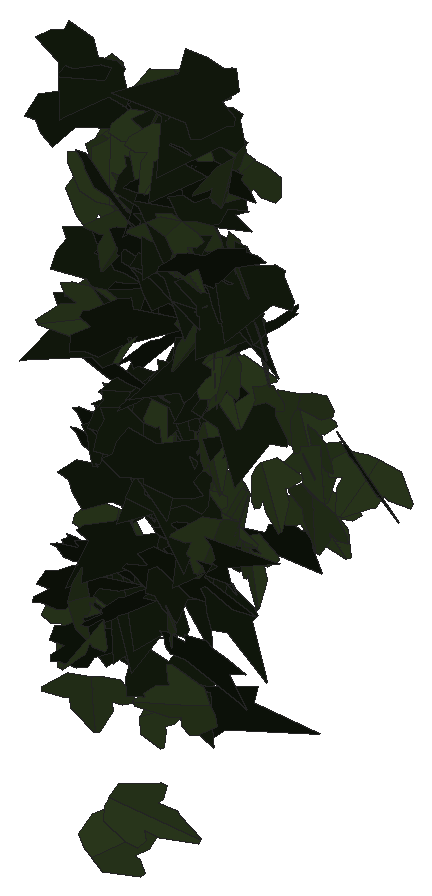
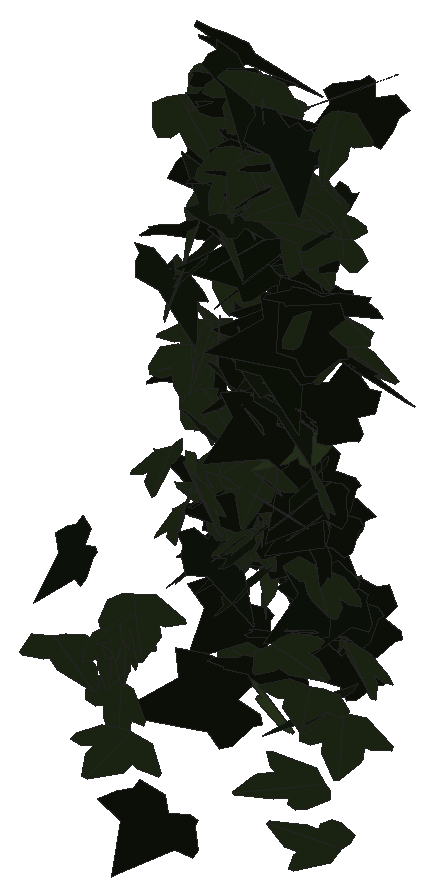
# SketchUp Ruby script. Lengths in inches.
U = 1.inch
M = Sketchup.active_model
def pt(a) = Geom::Point3d.new(a.map { |v| v * U })
def face(e, loops, mat)
  f = e.add_face(loops[0].map { |a| pt(a) })
  loops[1..].each { |l| e.add_face(l.map { |a| pt(a) }).erase! }
  f.material = f.back_material = mat if mat
  f
end
# faces: each face lists its corners as indices into pts; further lists are holes
def faces(e, pts, list, mat = nil) = list.each { |f| face(e, (f[0].is_a?(Array) ? f : [f]).map { |l| l.map { |i| pts[i] } }, mat) }
# xy, xz, yz: faces in a plane at the given z, y or x. An outline is a flat list of corners, or four numbers for a rectangle; further outlines are holes
def ring(l) = l.size == 4 ? [[l[0], l[1]], [l[2], l[1]], [l[2], l[3]], [l[0], l[3]]] : l.each_slice(2).to_a
def flat(e, list, mat, &to3) = list.each { |f| face(e, (f[0].is_a?(Array) ? f : [f]).map { |l| ring(l).map { |u, v| to3.(u, v) } }, mat) }
def xy(e, z, list, mat = nil) = flat(e, list, mat) { |x, y| [x, y, z] }
def xz(e, y, list, mat = nil) = flat(e, list, mat) { |x, z| [x, y, z] }
def yz(e, x, list, mat = nil) = flat(e, list, mat) { |y, z| [x, y, z] }
def lines(e, pts, list) = list.each { |a, b| e.add_line(pt(pts[a]), pt(pts[b])) }
# prism: a flat outline (further loops are holes) pulled along v
def prism(e, loops, v, mat = nil)
  f = face(e, loops, mat); d = Geom::Vector3d.new(v.map { |x| x * U })
  f.pushpull(f.normal.samedirection?(d) ? d.length : -d.length)
end
def box(e, o, s, mat = nil) = prism(e, [[o, [o[0] + s[0], o[1], o[2]], [o[0] + s[0], o[1] + s[1], o[2]], [o[0], o[1] + s[1], o[2]]]], [0, 0, s[2]], mat)
def at(x, y, z, deg = 0) = Geom::Transformation.translation(pt([x, y, z])) * Geom::Transformation.rotation(ORIGIN, Z_AXIS, deg.degrees)
def axes(o, x, y, z) = Geom::Transformation.new([*x, 0, *y, 0, *z, 0, *pt(o).to_a, 1])
def part(name) = M.definitions.add(name)
# library, detail: a bought-in or finely detailed component or shape, given as its bounding box
def library(name, o, s) = part(name).tap { |d| box(d.entities, o, s) }
def detail(e, o, s) = box(e.add_group.entities, o, s)
def put(e, d, t, mat = nil) = e.add_instance(d, t).tap { |i| i.material = mat if mat }
def group(e, t, mat = nil) = e.add_group.tap { |g| g.transformation = t; g.material = mat if mat }.entities
root = M.entities
M.materials.add("1026 AP 7946 SUNNY SIDE UP").color = [254, 231, 186]
M.materials.add("efeu1").color = [18, 25, 13]
M.materials.add("efeu2").color = [43, 57, 29]
c1 = part("ivyleaf_9")
p = [[1.54,2.16,1.25],[1.36,2.04,1.19],[-0.21,0.99,0.68],[-0.71,1.11,0.82],[-0.85,0.86,0.67],[-0.8,0.17,0.21],
  [-0.9,-0.01,0.1],[-0.67,-0.16,-0.02],[-0.08,-0.08,-0.05],[-0.03,-0.6,-0.4],[0.65,-0.88,-0.66],[0.83,-0.6,-0.49],
  [1.29,-0.42,-0.43],[1.8125,-0.07,-0.26],[1.21,0.44,0.15]]
faces(c1.entities,p,[[0,1,2,3,4,5,6,7,8,9,10,11,12,13,14]],"efeu1")
c2 = part("ivyleaf_10")
p = [[0,0.5,-0.03],[-0.0625,2.02,-0.43],[-0.19,2.01,-0.46],[-0.54,1.05,-0.29],[-0.52,0.625,-0.18],[-0.83,0.76,-0.28],
  [-1.16,0.64,-0.33],[-1.15,0.33,-0.24],[-0.77,-0.39,0.02],[-0.3,-0.51,0.16],[0.04,-0.48,0.23],[-0.02,2.01,-0.4375],
  [-0.06,2.01,-0.43],[0.04,-0.49,0.23],[0.67,-0.49,0.14],[1.38,0.36,-0.2],[1.375,0.51,-0.24],[0.81,0.65,-0.19],
  [0.62,0.59,-0.15],[0.6,1.09,-0.28],[0.5,1.23,-0.31]]
faces(c2.entities,p,[[0,1,2,3,4,5,6,7,8,9,10],[11,12,0,13,14,15,16,17,18,19,20]],"efeu2")
put(root,c1,axes([137.95,216.12,282.3],[0.42872,0.18972,0.0152],[0.02688,-0.00063,-0.34203],[-0.29788,0.27299,-0.00899]),"1026 AP 7946 SUNNY SIDE UP")
put(root,c1,axes([138.37,212.3,287.125],[-0.53188,0.04679,0.02114],[-0.04146,-0.04424,-0.34865],[-0.06861,-0.33596,0.04682]),"1026 AP 7946 SUNNY SIDE UP")
put(root,c2,axes([138.14,212.36,281.83],[-0.43427,-0.18901,-0.01024],[0.03781,-0.0195,-0.34353],[0.29512,-0.27563,0.02895]),"1026 AP 7946 SUNNY SIDE UP")
put(root,c2,axes([138.07,212.53,290.51],[-0.12663,-0.33819,-0.11167],[0.13132,0.08802,-0.35258],[0.54182,-0.10037,0.05935]),"1026 AP 7946 SUNNY SIDE UP")
put(root,c2,axes([138.08,212.2,282.89],[0.50514,-0.1536,0.01031],[-0.0055,-0.03245,-0.36566],[0.24207,0.3198,-0.02983]),"1026 AP 7946 SUNNY SIDE UP")
put(root,c1,axes([137.84,211.95,283.31],[0.26338,0.12076,0.27193],[0.34927,0.14163,-0.21168],[-0.29229,0.27805,-0.00792]),"1026 AP 7946 SUNNY SIDE UP")
put(root,c2,axes([137.98,213.19,282.72],[0.45525,0.13542,0.05238],[0.07469,0.01662,-0.32914],[-0.21439,0.29335,-0.00345]),"1026 AP 7946 SUNNY SIDE UP")
put(root,c2,axes([138.48,212.25,287.32],[0.34135,-0.05933,-0.31556],[-0.48308,0.02202,-0.22883],[0.08247,0.37451,-0.03428]),"1026 AP 7946 SUNNY SIDE UP")
put(root,c2,axes([138.14,212.86,285.62],[0.31499,-0.27005,0.01951],[0.03733,-0.00785,-0.34612],[0.42421,0.20121,0.01597]),"1026 AP 7946 SUNNY SIDE UP")
put(root,c1,axes([137.91,212.79,282.46],[0.31932,-0.22127,-0.13605],[-0.01575,0.15977,-0.2935],[0.40387,0.18118,0.09612]),"1026 AP 7946 SUNNY SIDE UP")
put(root,c1,axes([137.92,212.73,285.13],[0.52286,-0.01739,0.00805],[0.01101,-0.01733,-0.34269],[0.02794,0.33217,-0.01551]),"1026 AP 7946 SUNNY SIDE UP")
put(root,c2,axes([138.32,211.83,283.34],[-0.07815,0.13055,0.37213],[-0.2649,0.31909,-0.14111],[-0.54154,-0.17493,0.01532]),"1026 AP 7946 SUNNY SIDE UP")
put(root,c1,axes([138.15,212.42,283.77],[0.46242,0.10446,-0.11005],[-0.18167,0.00744,-0.31837],[-0.15001,0.313,0.04633]),"1026 AP 7946 SUNNY SIDE UP")
put(root,c1,axes([137.93,212.95,284.77],[0.03313,-0.03198,-0.33744],[0.4924,-0.09841,0.03009],[-0.15823,-0.31293,0.02299]),"1026 AP 7946 SUNNY SIDE UP")
put(root,c1,axes([138.18,212.37,290.85],[-0.24947,-0.28167,0.17286],[-0.01574,-0.18386,-0.32571],[0.51658,-0.14163,0.07356]),"1026 AP 7946 SUNNY SIDE UP")
put(root,c1,axes([137.97,212.4,283.72],[0.53065,0.096,0.08069],[0.10353,0.05169,-0.35975],[-0.1644,0.34245,0.03389]),"1026 AP 7946 SUNNY SIDE UP")
put(root,c1,axes([138.1,211.8125,290.58],[0.05421,-0.04347,-0.40499],[-0.10373,0.3882,-0.04795],[0.61281,0.06956,0.02771]),"1026 AP 7946 SUNNY SIDE UP")
put(root,c1,axes([137.8125,212.54,286.48],[0.30203,-0.16447,0.24232],[0.32031,-0.12285,-0.25956],[0.31963,0.27852,0.03113]),"1026 AP 7946 SUNNY SIDE UP")
put(root,c1,axes([138.04,212.86,285.14],[0.17389,-0.31256,-0.0502],[-0.00105,0.04951,-0.34088],[0.49698,0.10946,0.01684]),"1026 AP 7946 SUNNY SIDE UP")
put(root,c2,axes([138.22,212.67,284.09],[0.50889,-0.04895,-0.00527],[-0.00167,0.02524,-0.33609],[0.07733,0.32269,0.02743]),"1026 AP 7946 SUNNY SIDE UP")
put(root,c2,axes([138.32,212.57,287.58],[-0.33299,-0.27512,-0.01974],[0.04867,-0.00168,-0.35671],[0.43074,-0.2125,0.02505]),"1026 AP 7946 SUNNY SIDE UP")
put(root,c2,axes([138.45,213.16,283.18],[0.28779,0.15624,-0.22384],[-0.2585,-0.14343,-0.24874],[-0.33349,0.24601,-0.00036]),"1026 AP 7946 SUNNY SIDE UP")
put(root,c1,axes([138.09,211.94,282.59],[0.21475,0.11579,0.29698],[0.39679,0.1411,-0.18114],[-0.28327,0.28543,-0.02858]),"1026 AP 7946 SUNNY SIDE UP")
put(root,c1,axes([138.12,212.58,285.59],[0.52452,0.03111,0.03478],[0.05797,-0.03616,-0.34298],[-0.04267,0.33331,-0.03846]),"1026 AP 7946 SUNNY SIDE UP")
put(root,c1,axes([138.22,212.71,285.45],[0.52771,0.03995,-0.05944],[-0.0825,-0.046,-0.34613],[-0.07372,0.33745,-0.03811]),"1026 AP 7946 SUNNY SIDE UP")
put(root,c2,axes([138.39,212.41,289.0625],[0.61396,0.03855,0.04165],[-0.0709,0.05154,0.40045],[0.05144,-0.38912,0.05483]),"1026 AP 7946 SUNNY SIDE UP")
put(root,c1,axes([138.25,212.61,288.05],[-0.25066,-0.28804,-0.17007],[0.19697,0.11548,-0.33484],[0.48207,-0.19696,0.04838]),"1026 AP 7946 SUNNY SIDE UP")
put(root,c2,axes([138.03,212.48,288.91],[0.29702,-0.00979,0.32478],[0.49582,-0.00506,-0.1948],[0.01473,0.36753,0.00812]),"1026 AP 7946 SUNNY SIDE UP")
put(root,c1,axes([138.16,212.51,289.15],[0.26268,-0.29587,0.08312],[0.07745,-0.06673,-0.35028],[0.47667,0.17389,0.01111]),"1026 AP 7946 SUNNY SIDE UP")
put(root,c1,axes([138.31,212.92,285.22],[0.07404,-0.32159,0.06721],[0.00653,-0.06716,-0.33518],[0.51651,0.04695,-0.0054]),"1026 AP 7946 SUNNY SIDE UP")
put(root,c1,axes([138.68,212.74,290.34],[0.03034,0.35732,0.01618],[0.00274,0.0136,-0.36856],[-0.56225,0.01935,-0.00092]),"1026 AP 7946 SUNNY SIDE UP")
put(root,c2,axes([138.67,212.44,288.64],[-0.15481,-0.30808,0.14282],[-0.02385,-0.14204,-0.33291],[0.53181,-0.09605,0.02665]),"1026 AP 7946 SUNNY SIDE UP")
put(root,c1,axes([138.32,212.36,285.03],[-0.04851,-0.07724,-0.34935],[0.21188,0.31072,-0.08383],[0.50343,-0.13821,0.00162]),"1026 AP 7946 SUNNY SIDE UP")
put(root,c2,axes([138.32,212.69,289.54],[-0.34296,-0.11144,-0.30954],[0.45818,0.08049,-0.24872],[0.2075,-0.36193,0.03757]),"1026 AP 7946 SUNNY SIDE UP")
put(root,c1,axes([138.34,212.69,285.49],[0.35028,-0.24757,0.03355],[0.02972,-0.02869,-0.34323],[0.39181,0.22351,-0.00396]),"1026 AP 7946 SUNNY SIDE UP")
put(root,c1,axes([138.18,212.66,287.61],[0.50767,-0.04597,0.21665],[0.3158,-0.07338,-0.3342],[0.12292,0.3784,-0.03616]),"1026 AP 7946 SUNNY SIDE UP")
put(root,c1,axes([138.86,212.28,284.25],[0.07539,0.13523,-0.32928],[-0.11447,-0.31236,-0.14887],[-0.53472,0.08593,-0.01456]),"1026 AP 7946 SUNNY SIDE UP")
put(root,c2,axes([138.23,212.6875,289.01],[-0.06901,-0.02114,-0.39221],[0.58304,-0.09117,-0.03936],[-0.13894,-0.37211,0.02962]),"1026 AP 7946 SUNNY SIDE UP")
put(root,c1,axes([138.61,212.78,283.04],[-0.12573,-0.30723,0.0906],[-0.00156,-0.09221,-0.32684],[0.50325,-0.07704,0.02162]),"1026 AP 7946 SUNNY SIDE UP")
put(root,c1,axes([138.625,212.01,283.21],[0.23759,0.23325,0.22563],[0.16411,0.19148,-0.28488],[-0.47408,0.18318,0.01446]),"1026 AP 7946 SUNNY SIDE UP")
put(root,c2,axes([138.45,212.61,285.91],[0.37904,-0.2208,-0.07577],[0.31094,0.24967,-0.10484],[0.19178,0.03159,0.31974]),"1026 AP 7946 SUNNY SIDE UP")
put(root,c1,axes([138.75,212.77,283.14],[-0.3728,-0.22969,0.01212],[0.07047,-0.06452,-0.33095],[0.35482,-0.22852,0.07846]),"1026 AP 7946 SUNNY SIDE UP")
put(root,c1,axes([138.99,212.45,286.36],[-0.08541,0.32737,0.07438],[-0.07451,0.06302,-0.33952],[-0.52121,-0.06266,0.03635]),"1026 AP 7946 SUNNY SIDE UP")
put(root,c2,axes([138.83,215.62,284.72],[-0.35815,-0.23538,0.02415],[-0.00161,-0.03342,-0.33683],[0.37215,-0.22667,0.02179]),"1026 AP 7946 SUNNY SIDE UP")
put(root,c1,axes([138.45,212.56,287.36],[0.37956,0.12288,0.2599],[0.37019,0.09073,-0.27782],[-0.2383,0.33665,-0.01762]),"1026 AP 7946 SUNNY SIDE UP")
put(root,c1,axes([138.58,211.875,287.36],[0.1403,0.19253,-0.32],[0.05905,0.31433,0.21292],[0.57306,-0.07952,0.05641]),"1026 AP 7946 SUNNY SIDE UP")
put(root,c2,axes([138.72,216.03,283.02],[-0.41945,-0.14449,-0.14944],[0.26608,-0.02368,-0.29809],[0.17963,-0.30233,0.09259]),"1026 AP 7946 SUNNY SIDE UP")
put(root,c2,axes([138.625,212.01,279.82],[0.2186,0.09048,-0.3152],[0.3582,0.20632,0.17041],[0.35236,-0.26587,0.0223]),"1026 AP 7946 SUNNY SIDE UP")
put(root,c2,axes([138.91,212.98,285.42],[0.13341,0.25701,0.2001],[-0.0959,0.20864,-0.25769],[-0.49598,0.02878,0.10365]),"1026 AP 7946 SUNNY SIDE UP")
put(root,c1,axes([139.08,212.54,287.05],[-0.02278,0.3425,-0.06686],[0.01378,-0.06652,-0.3535],[-0.54854,-0.0159,-0.0061]),"1026 AP 7946 SUNNY SIDE UP")
put(root,c1,axes([138.82,212.51,285.95],[-0.16955,-0.30808,-0.09451],[0.05409,0.08329,-0.33574],[0.50176,-0.11309,0.00426]),"1026 AP 7946 SUNNY SIDE UP")
put(root,c2,axes([139.03,215.64,284.27],[-0.38712,0.21722,0.02043],[-0.09839,-0.04354,-0.3298],[-0.32838,-0.24303,0.07474]),"1026 AP 7946 SUNNY SIDE UP")
put(root,c1,axes([138.85,212.84,286.11],[0.2777,0.20587,0.20723],[0.21585,0.14562,-0.27848],[-0.39633,0.22356,-0.00647]),"1026 AP 7946 SUNNY SIDE UP")
put(root,c1,axes([139.09,212.99,285.125],[-0.47718,-0.06982,-0.11358],[0.19907,-0.09355,-0.29958],[0.04758,-0.30889,0.11434]),"1026 AP 7946 SUNNY SIDE UP")
put(root,c2,axes([139.21,212.78,285.32],[-0.48748,0.01167,0.12091],[-0.18501,-0.05053,-0.31549],[0.01118,-0.3276,0.05101]),"1026 AP 7946 SUNNY SIDE UP")
put(root,c1,axes([139.04,212.625,286.23],[-0.45145,-0.13408,-0.12],[0.19588,0.00382,-0.32292],[0.19797,-0.30953,0.04585]),"1026 AP 7946 SUNNY SIDE UP")
put(root,c2,axes([138.97,215.58,284.48],[0.01954,0.32821,-0.01036],[-0.00123,-0.0119,-0.33843],[-0.51641,0.01245,0.00041]),"1026 AP 7946 SUNNY SIDE UP")
put(root,c2,axes([139.0625,212.67,290.4],[0.14061,-0.3497,-0.01859],[0.06647,0.02724,-0.36843],[0.54641,0.08667,0.0496]),"1026 AP 7946 SUNNY SIDE UP")
put(root,c2,axes([139.17,215.56,283.35],[-0.47317,0.14296,0.05262],[-0.09923,-0.01661,-0.34062],[-0.21663,-0.30464,0.04109]),"1026 AP 7946 SUNNY SIDE UP")
put(root,c2,axes([139.04,212.72,285.86],[0.2255,0.29723,-0.03634],[-0.00697,-0.03887,-0.33996],[-0.47092,0.14291,-0.01237]),"1026 AP 7946 SUNNY SIDE UP")
put(root,c1,axes([138.64,212.36,288.18],[0.24456,-0.05448,0.33598],[0.48034,-0.11514,-0.17041],[0.20022,0.34278,-0.00156]),"1026 AP 7946 SUNNY SIDE UP")
put(root,c1,axes([139.49,212.82,286.11],[-0.10643,-0.13238,-0.31536],[-0.27789,-0.24976,0.15044],[-0.44346,0.18828,-0.01858]),"1026 AP 7946 SUNNY SIDE UP")
put(root,c1,axes([138.98,212.36,285.83],[-0.10527,-0.34112,-0.10654],[0.07399,0.09387,-0.35649],[0.55469,-0.07726,0.02733]),"1026 AP 7946 SUNNY SIDE UP")
put(root,c1,axes([139.42,212.62,286.78],[-0.37173,0.2263,-0.09427],[0.04104,-0.10497,-0.33286],[-0.3824,-0.23126,0.05592]),"1026 AP 7946 SUNNY SIDE UP")
put(root,c2,axes([139.15,212.36,290.16],[0.55968,-0.02919,-0.00552],[-0.01155,-0.02621,-0.36704],[0.04516,0.35501,-0.02545]),"1026 AP 7946 SUNNY SIDE UP")
put(root,c2,axes([139.17,212.71,284.38],[-0.04591,0.28419,-0.1655],[0.0064,-0.16258,-0.29505],[-0.51453,-0.02738,0.0111]),"1026 AP 7946 SUNNY SIDE UP")
put(root,c1,axes([139.08,212.52,289.31],[-0.04327,-0.35443,0.02912],[-0.0005,-0.03035,-0.3664],[0.55933,-0.02744,0.00192]),"1026 AP 7946 SUNNY SIDE UP")
put(root,c2,axes([139.22,215.56,284.12],[-0.23275,-0.29253,-0.01229],[0.11378,-0.02541,-0.32869],[0.44597,-0.14618,0.07744]),"1026 AP 7946 SUNNY SIDE UP")
put(root,c2,axes([139.33,212.66,289.47],[-0.2041,-0.31445,0.09645],[-0.01348,-0.09931,-0.34977],[0.51652,-0.12684,0.02898]),"1026 AP 7946 SUNNY SIDE UP")
put(root,c2,axes([139.19,212.875,284.45],[0.12463,0.31723,-0.0542],[-0.00447,-0.05534,-0.337],[-0.50607,0.07861,-0.01037]),"1026 AP 7946 SUNNY SIDE UP")
put(root,c1,axes([139.48,212.47,285.36],[-0.49738,-0.10483,0.00487],[0.00798,-0.03214,-0.34189],[0.16486,-0.31472,0.03123]),"1026 AP 7946 SUNNY SIDE UP")
put(root,c2,axes([139.14,212.59,286.07],[0.01346,-0.31323,0.15881],[0.29861,-0.12685,-0.27398],[0.46209,0.09109,0.17243]),"1026 AP 7946 SUNNY SIDE UP")
put(root,c1,axes([139.11,212.44,288.21],[0.24839,-0.25169,-0.19586],[-0.08118,0.18754,-0.30113],[0.48791,0.15933,0.04961]),"1026 AP 7946 SUNNY SIDE UP")
put(root,c2,axes([139.04,212.47,281.69],[0.15798,-0.26625,-0.18959],[0.28173,-0.11301,0.27077],[-0.42221,-0.17503,0.10974]),"1026 AP 7946 SUNNY SIDE UP")
put(root,c2,axes([139.27,212.71,290.75],[-0.47222,-0.18249,-0.08389],[0.18001,-0.03877,-0.35011],[0.25674,-0.30846,0.09118]),"1026 AP 7946 SUNNY SIDE UP")
put(root,c1,axes([139.31,212.59,288.93],[-0.23888,-0.29224,0.12369],[-0.03385,-0.12516,-0.33798],[0.49663,-0.1491,0.03645]),"1026 AP 7946 SUNNY SIDE UP")
put(root,c2,axes([139,211.99,280.55],[0.13058,0.10916,0.33207],[0.37123,0.21961,-0.13826],[-0.38412,0.24934,-0.02074]),"1026 AP 7946 SUNNY SIDE UP")
put(root,c1,axes([139.52,212.38,289.59],[0.00696,0.25924,-0.284],[-0.0102,-0.27708,-0.26872],[-0.59663,0.00776,0.00128]),"1026 AP 7946 SUNNY SIDE UP")
put(root,c2,axes([139.61,212.62,284.46],[-0.44664,-0.01544,0.1887],[-0.26993,-0.09869,-0.28326],[0.10373,-0.32331,0.07538]),"1026 AP 7946 SUNNY SIDE UP")
put(root,c1,axes([139.18,212.95,284.48],[0.09888,-0.32337,-0.01361],[-0.0212,0.00896,-0.33912],[0.50835,0.06327,-0.01149]),"1026 AP 7946 SUNNY SIDE UP")
put(root,c1,axes([139.8,212.56,290],[-0.06682,0.05866,0.3661],[-0.5158,0.14066,-0.06357],[-0.23262,-0.32874,0.03579]),"1026 AP 7946 SUNNY SIDE UP")
put(root,c1,axes([139.14,212.88,284.43],[0.27869,-0.28014,-0.00628],[0.02396,0.01496,-0.34074],[0.43989,0.17666,0.02253]),"1026 AP 7946 SUNNY SIDE UP")
put(root,c1,axes([139.01,212.69,284.69],[0.11314,-0.00175,-0.34027],[0.40087,0.2152,0.0573],[0.33018,-0.26068,0.04702]),"1026 AP 7946 SUNNY SIDE UP")
put(root,c1,axes([139.11,212.55,288.09],[-0.02082,-0.31941,0.16766],[0.27102,-0.15013,-0.2868],[0.49572,0.06867,0.16384]),"1026 AP 7946 SUNNY SIDE UP")
put(root,c2,axes([139.2,212.83,285.875],[-0.06909,0.01699,-0.34545],[0.23374,-0.30235,-0.0376],[-0.47354,-0.15172,0.03184]),"1026 AP 7946 SUNNY SIDE UP")
put(root,c1,axes([139.59,212.45,290.67],[0.05406,0.33089,0.17726],[-0.01497,0.17164,-0.3408],[-0.58489,0.02619,0.0251]),"1026 AP 7946 SUNNY SIDE UP")
put(root,c1,axes([139.21,212.57,282.42],[-0.12203,-0.24703,-0.21194],[0.23842,0.15694,-0.25388],[0.44414,-0.15212,0.07806]),"1026 AP 7946 SUNNY SIDE UP")
put(root,c1,axes([139.06,212.76,288.32],[0.45457,-0.16439,0.11323],[0.16631,-0.03789,-0.34231],[0.26368,0.30729,0.02071]),"1026 AP 7946 SUNNY SIDE UP")
put(root,c2,axes([139.29,212.61,288.56],[0.29299,-0.18472,0.23937],[0.22948,-0.1833,-0.27055],[0.40792,0.23579,-0.01973]),"1026 AP 7946 SUNNY SIDE UP")
put(root,c1,axes([139.25,212.84,283.65],[0.1178,-0.31652,0.05664],[0.01076,-0.05672,-0.33536],[0.50553,0.07497,-0.00606]),"1026 AP 7946 SUNNY SIDE UP")
put(root,c1,axes([139.36,212.83,286.37],[-0.09489,-0.33505,0.00152],[0.00447,-0.00394,-0.35072],[0.52684,-0.06031,0.00325]),"1026 AP 7946 SUNNY SIDE UP")
put(root,c2,axes([139.87,212.27,282.21],[-0.19899,0.03952,0.31173],[-0.46781,-0.08782,-0.11697],[0.10519,-0.3158,0.06952]),"1026 AP 7946 SUNNY SIDE UP")
put(root,c1,axes([139.87,212.91,285.77],[-0.3218,0.24293,0.1032],[-0.18038,0.02976,-0.32004],[-0.37082,-0.2253,0.06612]),"1026 AP 7946 SUNNY SIDE UP")
put(root,c2,axes([139.28,212.4,283.33],[-0.15977,0.03682,0.3372],[0.37755,-0.22588,0.10171],[0.35406,0.25749,0.0437]),"1026 AP 7946 SUNNY SIDE UP")
put(root,c2,axes([139.57,212.23,290.18],[0.43417,0.17583,-0.14784],[-0.17588,-0.09302,-0.33733],[-0.31166,0.29744,-0.01558]),"1026 AP 7946 SUNNY SIDE UP")
put(root,c1,axes([139.42,212.24,284.07],[0.22033,-0.0507,-0.34839],[-0.21983,0.32473,-0.10802],[0.49022,0.1684,0.10815]),"1026 AP 7946 SUNNY SIDE UP")
put(root,c2,axes([139.81,212.89,286.1],[-0.435,-0.04651,0.18369],[-0.26319,-0.07222,-0.28694],[0.12214,-0.32125,0.0359]),"1026 AP 7946 SUNNY SIDE UP")
put(root,c2,axes([139.67,212.25,288.95],[-0.41455,-0.2335,0.04107],[-0.0116,-0.05349,-0.36134],[0.37265,-0.26142,0.03444]),"1026 AP 7946 SUNNY SIDE UP")
put(root,c1,axes([139.45,212.43,285.12],[-0.11277,-0.34231,-0.01894],[0.02792,0.01306,-0.35991],[0.53814,-0.07241,0.0147]),"1026 AP 7946 SUNNY SIDE UP")
put(root,c1,axes([139.29,212,285.41],[-0.10888,0.01276,0.35933],[0.54597,0.03792,0.06982],[-0.05464,0.3535,-0.01837]),"1026 AP 7946 SUNNY SIDE UP")
put(root,c2,axes([139.57,212.64,289.49],[-0.30714,-0.31227,-0.15716],[0.15691,0.11511,-0.37812],[0.52219,-0.21826,0.02118]),"1026 AP 7946 SUNNY SIDE UP")
put(root,c1,axes([139.89,212.51,286.51],[-0.13854,0.29422,0.1563],[-0.12218,0.13248,-0.31383],[-0.50475,-0.11282,0.03306]),"1026 AP 7946 SUNNY SIDE UP")
put(root,c2,axes([139.88,212.625,288.55],[0.0768,-0.13973,-0.38216],[-0.29117,0.32153,-0.14833],[0.54979,0.1898,-0.02517]),"1026 AP 7946 SUNNY SIDE UP")
put(root,c1,axes([139.52,212.77,289.47],[-0.21674,-0.3193,-0.04678],[0.0789,0.02558,-0.35625],[0.50055,-0.14229,0.0359]),"1026 AP 7946 SUNNY SIDE UP")
put(root,c1,axes([139.49,212.57,288.28],[-0.06902,-0.32833,0.11074],[0.01061,-0.11103,-0.34126],[0.54405,-0.03949,0.02071]),"1026 AP 7946 SUNNY SIDE UP")
put(root,c2,axes([139.38,212.19,288.87],[-0.37094,0.05385,-0.27402],[0.34115,-0.17492,-0.23547],[-0.25712,-0.30978,0.08289]),"1026 AP 7946 SUNNY SIDE UP")
put(root,c1,axes([139.77,212.53,290.24],[-0.42593,-0.23269,0.03566],[-0.02435,-0.03705,-0.36764],[0.36942,-0.27073,0.01688]),"1026 AP 7946 SUNNY SIDE UP")
put(root,c1,axes([139.31,212.11,284.06],[0.49685,0.07085,0.16989],[0.26722,-0.01318,-0.3305],[-0.089,0.356,-0.04388]),"1026 AP 7946 SUNNY SIDE UP")
put(root,c1,axes([139.9,212.77,284.03],[-0.11131,0.30814,-0.10871],[0.00089,-0.10965,-0.32551],[-0.51304,-0.06704,0.02302]),"1026 AP 7946 SUNNY SIDE UP")
put(root,c1,axes([139.97,212.2,287.17],[-0.43772,0.19566,-0.04724],[0.03571,-0.04912,-0.34973],[-0.31437,-0.27801,0.02606]),"1026 AP 7946 SUNNY SIDE UP")
put(root,c1,axes([140.15,212.34,290.95],[-0.44921,0.12123,0.18913],[-0.29121,0.02782,-0.31685],[-0.18505,-0.33807,0.0395]),"1026 AP 7946 SUNNY SIDE UP")
put(root,c1,axes([139.33,212.85,288.82],[0.01413,-0.33715,0.08525],[0.5343,-0.00934,-0.07553],[0.11527,0.08463,0.33965]),"1026 AP 7946 SUNNY SIDE UP")
put(root,c1,axes([139.83,212.55,290.63],[-0.43251,-0.22433,0.014],[0.00201,-0.02505,-0.36521],[0.3535,-0.27432,0.01921]),"1026 AP 7946 SUNNY SIDE UP")
put(root,c2,axes([139.8,215.85,283.96],[0.47361,0.1062,-0.12193],[-0.17485,-0.04236,-0.32925],[-0.17973,0.32106,-0.00099]),"1026 AP 7946 SUNNY SIDE UP")
put(root,c2,axes([139.77,212.85,287.02],[-0.07543,0.28886,-0.17674],[0.00771,-0.17434,-0.30194],[-0.52954,-0.04368,0.02078]),"1026 AP 7946 SUNNY SIDE UP")
put(root,c2,axes([139.85,212.85,286.96],[-0.01859,-0.2283,-0.26073],[0.05781,0.2496,-0.23347],[0.53129,-0.03515,0.01628]),"1026 AP 7946 SUNNY SIDE UP")
put(root,c1,axes([139.96,212.2,290.05],[0.35908,0.16233,-0.23264],[-0.31246,-0.11089,-0.28861],[-0.30764,0.3021,0.02159]),"1026 AP 7946 SUNNY SIDE UP")
put(root,c2,axes([139.49,212.72,284.67],[-0.09946,-0.00164,-0.34231],[0.49064,-0.11655,-0.06128],[-0.17958,-0.31752,0.02215]),"1026 AP 7946 SUNNY SIDE UP")
put(root,c1,axes([139.59,212.88,286.53],[0.04167,-0.03376,0.3462],[0.18895,-0.31429,-0.0441],[0.49665,0.12241,-0.01227]),"1026 AP 7946 SUNNY SIDE UP")
put(root,c1,axes([139.91,212.63,284.6],[-0.24422,-0.26497,0.12944],[-0.09555,-0.11175,-0.31704],[0.45213,-0.16674,0.00292]),"1026 AP 7946 SUNNY SIDE UP")
put(root,c2,axes([139.9375,212.39,287.6875],[0.0148,-0.27851,0.21865],[0.01935,-0.21351,-0.2883],[0.55177,0.01496,0.00425]),"1026 AP 7946 SUNNY SIDE UP")
put(root,c2,axes([139.93,212.98,284.96],[0.37653,-0.22715,-0.02413],[-0.04382,0.00274,-0.33955],[0.35617,0.24047,-0.01626]),"1026 AP 7946 SUNNY SIDE UP")
put(root,c1,axes([139.72,212.31,282.99],[0.52653,0.01339,-0.04396],[-0.06476,-0.03479,-0.34378],[-0.02771,0.33578,-0.03188]),"1026 AP 7946 SUNNY SIDE UP")
put(root,c2,axes([139.88,212.55,285.92],[-0.02551,0.33076,-0.03021],[0.00173,-0.03119,-0.34134],[-0.5224,-0.01626,0.00035]),"1026 AP 7946 SUNNY SIDE UP")
put(root,c1,axes([139.59,212.72,281.875],[0.42556,0.12785,0.27251],[0.40618,0.06571,-0.30546],[-0.2179,0.37218,-0.03718]),"1026 AP 7946 SUNNY SIDE UP")
put(root,c2,axes([140.16,212.85,286.6],[-0.46878,-0.14825,0.02842],[-0.01606,-0.04299,-0.34149],[0.23682,-0.29638,0.03311]),"1026 AP 7946 SUNNY SIDE UP")
put(root,c1,axes([139.63,212.24,284.43],[0.38949,0.10248,-0.23601],[0.3069,0.12498,0.27503],[0.2494,-0.31383,0.03014]),"1026 AP 7946 SUNNY SIDE UP")
put(root,c2,axes([140.11,212.53,287.07],[0.43097,-0.21632,0.00298],[-0.02143,-0.02391,-0.35875],[0.33952,0.27307,-0.02643]),"1026 AP 7946 SUNNY SIDE UP")
put(root,c2,axes([140.18,212.27,284.83],[-0.19619,-0.29404,0.09826],[0.01119,-0.10733,-0.3262],[0.48676,-0.11605,0.04711]),"1026 AP 7946 SUNNY SIDE UP")
put(root,c2,axes([140.42,212.625,289.96],[-0.47844,-0.05884,0.18016],[-0.24894,-0.0912,-0.31531],[0.14999,-0.33907,0.05136]),"1026 AP 7946 SUNNY SIDE UP")
put(root,c2,axes([140.125,212.83,284.94],[0.28728,-0.26273,0.10176],[0.08049,-0.08651,-0.3301],[0.43479,0.18961,-0.00613]),"1026 AP 7946 SUNNY SIDE UP")
put(root,c1,axes([140.28,211.95,288.92],[0.22927,0.30673,-0.07845],[-0.05109,-0.07081,-0.35029],[-0.49498,0.14938,-0.00019]),"1026 AP 7946 SUNNY SIDE UP")
put(root,c2,axes([140.23,212.6,288.61],[-0.28086,0.31232,0.0477],[-0.05645,0.03072,-0.37011],[-0.49283,-0.18151,0.01521]),"1026 AP 7946 SUNNY SIDE UP")
put(root,c1,axes([140.2,212.63,287.92],[-0.27713,-0.26097,0.16354],[-0.00336,-0.18381,-0.31193],[0.48151,-0.15149,0.09194]),"1026 AP 7946 SUNNY SIDE UP")
put(root,c2,axes([140.125,212.58,286.94],[0.26683,0.29569,0.03564],[0.02355,0.02935,-0.35104],[-0.46722,0.17035,0.00266]),"1026 AP 7946 SUNNY SIDE UP")
put(root,c1,axes([140.08,212.64,288.04],[0.2541,-0.30579,-0.04055],[-0.0142,0.03777,-0.35594],[0.48424,0.16156,0.01084]),"1026 AP 7946 SUNNY SIDE UP")
put(root,c1,axes([140.13,212.55,283.69],[0.19501,-0.30228,-0.06911],[-0.04956,0.0577,-0.33618],[0.48376,0.12777,-0.00658]),"1026 AP 7946 SUNNY SIDE UP")
put(root,c1,axes([140.3125,212.75,286.39],[-0.19078,-0.31228,0.0179],[0.00511,-0.0218,-0.34508],[0.49193,-0.12088,0.01053]),"1026 AP 7946 SUNNY SIDE UP")
put(root,c2,axes([140.46,212.19,290.19],[-0.0419,-0.36789,-0.0688],[0.00099,0.06481,-0.37959],[0.58734,-0.02635,-0.00427]),"1026 AP 7946 SUNNY SIDE UP")
put(root,c1,axes([140.37,212.79,288.42],[-0.29525,-0.29155,0.04037],[0.03392,-0.06194,-0.35369],[0.46167,-0.18191,0.0518]),"1026 AP 7946 SUNNY SIDE UP")
put(root,c1,axes([140.24,214.9,284.79],[0.42444,-0.15168,-0.12881],[-0.1784,0.05144,-0.31851],[0.25136,0.29264,-0.00855]),"1026 AP 7946 SUNNY SIDE UP")
put(root,c1,axes([140.66,212.67,287.65],[-0.068,0.33486,0.07375],[-0.07316,0.06383,-0.34535],[-0.53282,-0.0515,0.038]),"1026 AP 7946 SUNNY SIDE UP")
put(root,c2,axes([140.36,213.09,285.28],[0.05723,0.33003,0.015],[-0.00235,0.01293,-0.34197],[-0.51932,0.03631,0.0032]),"1026 AP 7946 SUNNY SIDE UP")
put(root,c2,axes([140.37,212.77,284.37],[-0.02421,0.32622,-0.07656],[0.00071,-0.07623,-0.33687],[-0.52674,-0.01509,0.00306]),"1026 AP 7946 SUNNY SIDE UP")
put(root,c2,axes([140.46,212.76,287.62],[-0.22565,0.31304,-0.04688],[-0.00019,-0.05197,-0.35437],[-0.4978,-0.14188,0.02139]),"1026 AP 7946 SUNNY SIDE UP")
